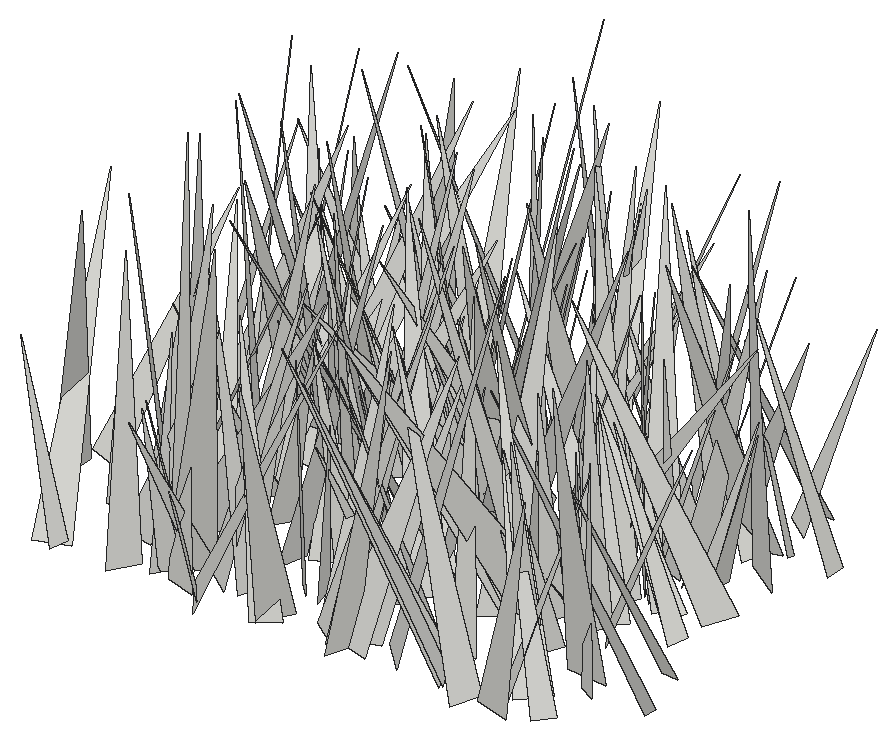
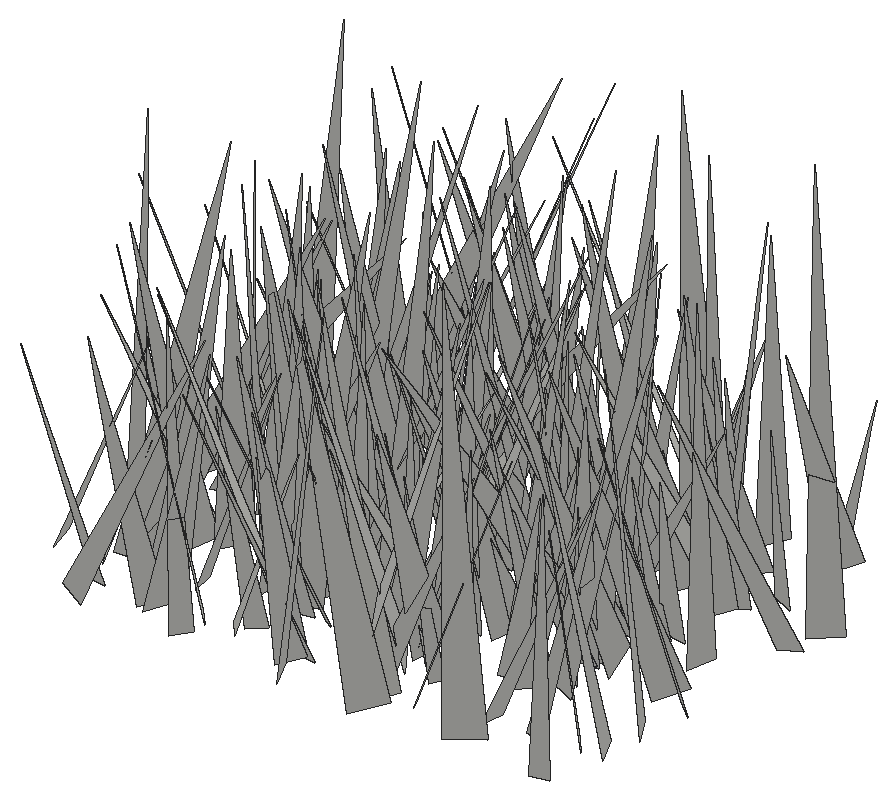
# SketchUp Ruby script. Lengths in inches.
U = 1.inch
M = Sketchup.active_model
def pt(a) = Geom::Point3d.new(a.map { |v| v * U })
def face(e, loops, mat)
  f = e.add_face(loops[0].map { |a| pt(a) })
  loops[1..].each { |l| e.add_face(l.map { |a| pt(a) }).erase! }
  f.material = f.back_material = mat if mat
  f
end
# faces: each face lists its corners as indices into pts; further lists are holes
def faces(e, pts, list, mat = nil) = list.each { |f| face(e, (f[0].is_a?(Array) ? f : [f]).map { |l| l.map { |i| pts[i] } }, mat) }
# xy, xz, yz: faces in a plane at the given z, y or x. An outline is a flat list of corners, or four numbers for a rectangle; further outlines are holes
def ring(l) = l.size == 4 ? [[l[0], l[1]], [l[2], l[1]], [l[2], l[3]], [l[0], l[3]]] : l.each_slice(2).to_a
def flat(e, list, mat, &to3) = list.each { |f| face(e, (f[0].is_a?(Array) ? f : [f]).map { |l| ring(l).map { |u, v| to3.(u, v) } }, mat) }
def xy(e, z, list, mat = nil) = flat(e, list, mat) { |x, y| [x, y, z] }
def xz(e, y, list, mat = nil) = flat(e, list, mat) { |x, z| [x, y, z] }
def yz(e, x, list, mat = nil) = flat(e, list, mat) { |y, z| [x, y, z] }
def lines(e, pts, list) = list.each { |a, b| e.add_line(pt(pts[a]), pt(pts[b])) }
# prism: a flat outline (further loops are holes) pulled along v
def prism(e, loops, v, mat = nil)
  f = face(e, loops, mat); d = Geom::Vector3d.new(v.map { |x| x * U })
  f.pushpull(f.normal.samedirection?(d) ? d.length : -d.length)
end
def box(e, o, s, mat = nil) = prism(e, [[o, [o[0] + s[0], o[1], o[2]], [o[0] + s[0], o[1] + s[1], o[2]], [o[0], o[1] + s[1], o[2]]]], [0, 0, s[2]], mat)
def at(x, y, z, deg = 0) = Geom::Transformation.translation(pt([x, y, z])) * Geom::Transformation.rotation(ORIGIN, Z_AXIS, deg.degrees)
def axes(o, x, y, z) = Geom::Transformation.new([*x, 0, *y, 0, *z, 0, *pt(o).to_a, 1])
def part(name) = M.definitions.add(name)
# library, detail: a bought-in or finely detailed component or shape, given as its bounding box
def library(name, o, s) = part(name).tap { |d| box(d.entities, o, s) }
def detail(e, o, s) = box(e.add_group.entities, o, s)
def put(e, d, t, mat = nil) = e.add_instance(d, t).tap { |i| i.material = mat if mat }
def group(e, t, mat = nil) = e.add_group.tap { |g| g.transformation = t; g.material = mat if mat }.entities
root = M.entities
c1 = part("fur_instance\#9")
p = [[0.8125,0,1.79],[0.67,-0.02,1.48],[0,-0.11,0],[0,0.11,0]]
faces(c1.entities,p,[[0,1,2,3]])
put(root,c1,axes([515.01,5.77,-21.86],[4.57924,-4.33247,0.58798],[-4.22206,-4.60304,-1.03525],[-1.13589,-0.35667,6.21836]))
put(root,c1,axes([521.93,6.4375,-21.86],[-6.83596,-2.73328,0.53057],[-2.58478,6.75268,1.48423],[1.035,-1.18879,7.21098]))
put(root,c1,axes([524.83,5.37,-21.86],[0.54307,-5.39112,1.14857],[-5.29865,-0.1925,1.60174],[1.51911,1.25582,5.17624]))
put(root,c1,axes([522.02,6.35,-21.86],[-5.72076,-3.26575,0.35826],[-3.1922,5.6955,0.94426],[0.77675,-0.64548,6.51924]))
put(root,c1,axes([510.13,6.12,-21.86],[2.18541,-3.04998,0.78828],[-3.02604,-2.29919,-0.50659],[-0.87571,0.3334,3.71777]))
put(root,c1,axes([511.02,6.96,-21.86],[1.51991,-3.61395,0.26794],[-3.4425,-1.53065,-1.11749],[-1.13207,-0.1975,3.75792]))
put(root,c1,axes([505.96,5.14,-21.86],[-3.79892,0.58903,0.61511],[0.5899,3.84804,-0.04166],[0.61427,-0.05255,3.84409]))
put(root,c1,axes([518.15,5.42,-21.86],[6.14943,-1.42717,1.61929],[-1.52874,-6.3314,0.22535],[-1.52376,0.59247,6.30885]))
put(root,c1,axes([510.14,7.22,-21.86],[6.18232,-5.30847,0.7026],[-5.32058,-6.21081,-0.10875],[-0.60412,0.37485,8.14795]))
put(root,c1,axes([511.93,5.12,-21.86],[5.9079,4.20697,0.32991],[4.15488,-5.69984,-1.72033],[0.73785,-1.5887,7.04573]))
put(root,c1,axes([512.08,5.14,-21.86],[-3.12705,-1.8127,0.50032],[-1.87769,2.95706,-1.02213],[-0.10232,1.13341,3.46693]))
put(root,c1,axes([508.7,5.31,-21.86],[-5.0872,2.66073,2.45988],[2.85923,5.55214,-0.09239],[2.22604,-1.05084,5.74025]))
put(root,c1,axes([514.94,5.33,-21.86],[-2.01026,5.06538,1.49078],[5.275,1.85579,0.80751],[-0.23431,-1.67916,5.38954]))
put(root,c1,axes([523.74,5.29,-21.86],[-6.69944,1.03913,0.45559],[1.00559,6.70154,-0.49804],[0.5255,0.42362,6.76123]))
put(root,c1,axes([517.66,5.93,-21.86],[5.24089,-0.83273,1.62957],[-1.05437,-5.41429,0.62423],[-1.49573,0.89885,5.2698]))
put(root,c1,axes([518.24,5.71,-21.86],[0.11042,6.13884,2.00494],[6.14565,0.51615,-1.91884],[1.98398,-1.94051,5.83229]))
put(root,c1,axes([503.14,9.33,-21.86],[8.00988,-2.00577,0.3429],[-1.833,-7.71682,-2.32157],[-0.88363,-2.17404,7.92412]))
put(root,c1,axes([511.07,5.46,-21.86],[2.99088,7.34321,2.70362],[7.47912,-3.53374,1.32409],[-2.30112,-1.94104,7.81761]))
put(root,c1,axes([526.625,5.99,-21.86],[-1.36293,4.52681,0.55653],[4.38086,1.13777,1.47406],[-1.26877,-0.93423,4.49185]))
put(root,c1,axes([509.84,5.78,-21.86],[-4.10668,0.43412,1.0008],[0.12519,4.05996,-1.24738],[1.0837,1.17608,3.93666]))
put(root,c1,axes([524.67,7.86,-21.86],[1.7038,-4.78318,1.39426],[-4.94528,-1.80274,-0.14134],[-0.60574,1.26373,5.0756]))
put(root,c1,axes([511.69,6.65,-21.86],[3.29943,5.39851,1.49465],[5.593,-3.07886,-1.22601],[0.31023,-1.9081,6.20701]))
put(root,c1,axes([525.93,9.21,-21.86],[0.64901,-7.30772,0.94418],[-7.33385,-0.54888,0.79295],[0.71332,1.00569,7.2935]))
put(root,c1,axes([524.82,5.97,-21.86],[3.07177,3.42083,0.35758],[3.42072,-3.08846,0.16062],[-0.35863,-0.15826,4.59478]))
put(root,c1,axes([519.84,6.17,-21.86],[5.42391,5.6075,1.42758],[5.74422,-5.4537,-0.40246],[-0.69711,-1.3092,7.79108]))
put(root,c1,axes([507.74,7.23,-21.86],[1.80806,-4.3936,1.6396],[-4.55829,-1.23367,1.72079],[1.10181,2.10605,4.4285]))
put(root,c1,axes([515.34,8,-21.86],[3.69206,0.52175,1.19179],[0.74035,-3.79133,-0.63373],[-1.0698,-0.8231,3.6745]))
put(root,c1,axes([520.88,7.52,-21.86],[-4.50374,-2.5863,0.2222],[-2.55985,4.35118,-1.23954],[-0.43072,1.18335,5.04343]))
put(root,c1,axes([522.21,11.63,-21.86],[4.91107,-6.51993,1.1851],[-5.42781,-4.80392,-3.93621],[-3.80168,-1.5638,7.15082]))
put(root,c1,axes([513.12,6.66,-21.86],[-5.72971,0.10944,0.75393],[-0.02545,5.68949,-1.01935],[0.7614,1.01378,5.63937]))
put(root,c1,axes([517.03,5.94,-21.86],[4.48947,6.23838,0.89691],[6.27438,-4.52789,0.08708],[-0.59503,-0.67674,7.68539]))
put(root,c1,axes([507.99,8.89,-21.86],[-4.21383,-5.23135,2.06774],[-5.35043,4.52497,0.54449],[1.7365,1.24763,6.69529]))
put(root,c1,axes([525.42,6.91,-21.86],[-3.60307,5.2202,0.86904],[5.28801,3.51043,0.83765],[-0.20649,-1.18922,6.28736]))
put(root,c1,axes([517.56,9.05,-21.86],[0.6602,-3.48398,0.63366],[-3.31771,-0.83389,-1.12823],[-1.23791,0.37685,3.36171]))
put(root,c1,axes([505.6875,5.11,-21.86],[-5.02723,4.35262,0.08247],[4.19421,4.87628,-1.68986],[1.1665,1.22544,6.43138]))
put(root,c1,axes([514.53,7.9375,-21.86],[2.78644,2.89477,1.9564],[3.12581,-3.18339,0.25829],[-1.56092,-1.20736,4.00964]))
put(root,c1,axes([516.08,8.74,-21.86],[2.18387,-4.44969,1.85832],[-4.59717,-2.53702,-0.67228],[-1.45572,1.33648,4.91091]))
put(root,c1,axes([518.57,6.35,-21.86],[-3.94538,2.89092,1.6801],[2.22143,4.20848,-2.02488],[2.49909,0.82308,4.45234]))
put(root,c1,axes([516.7,6.97,-21.86],[0.1573,5.82785,1.1486],[5.93788,-0.12389,-0.18455],[0.15705,-1.15268,5.82705]))
put(root,c1,axes([516.33,7.68,-21.86],[6.01682,-1.89651,1.60783],[-2.22,-5.99358,1.23799],[-1.11958,1.69241,6.18597]))
put(root,c1,axes([526.65,8.32,-21.86],[2.05844,3.54151,1.67651],[3.74882,-2.33096,0.32115],[-1.13989,-1.27062,4.08367]))
put(root,c1,axes([523.8,9.9,-21.86],[3.25434,-3.10316,1.28908],[-2.93626,-3.49873,-1.00964],[-1.63392,0.10675,4.38189]))
put(root,c1,axes([508.94,9.32,-21.86],[3.69144,-5.31541,0.62902],[-5.0613,-3.21782,2.51095],[1.74141,1.9152,5.96452]))
put(root,c1,axes([521.02,11.38,-21.86],[-6.06549,-1.51995,0.44377],[-1.27134,5.72216,2.22212],[0.94386,-2.06007,5.84487]))
put(root,c1,axes([529.18,8.63,-21.86],[-3.79929,-4.93063,0.76728],[-4.2284,2.66909,-3.78564],[-2.64961,2.81057,4.94112]))
put(root,c1,axes([505.8,8.41,-21.86],[0.89714,3.83975,1.01573],[3.88067,-1.06922,0.61438],[-0.84607,-0.83267,3.89501]))
put(root,c1,axes([506.81,9.65,-21.86],[1.60896,-4.17155,1.4473],[-4.41412,-1.4813,0.63763],[0.1098,1.57772,4.42538]))
put(root,c1,axes([521.68,7.73,-21.86],[1.15539,6.15443,1.22459],[6.01284,-1.44203,1.57415],[-1.79512,-0.86897,6.06086]))
put(root,c1,axes([515.49,9.5,-21.86],[2.89079,5.81329,3.19782],[6.3896,-3.37876,0.3661],[-1.787,-2.67707,6.48205]))
put(root,c1,axes([528.125,11.05,-21.86],[-1.33885,-4.31341,0.19295],[-4.24788,1.27969,-0.86785],[-0.77346,0.43835,4.43226]))
put(root,c1,axes([522.77,10.72,-21.86],[-7.92829,-1.68885,1.19775],[-1.65667,8.01779,0.33921],[1.24187,-0.08605,8.09907]))
put(root,c1,axes([519.47,10.6,-21.86],[-4.42248,-6.55022,0.11235],[-5.68971,3.77318,-3.9833],[-3.24733,2.30957,6.8262]))
put(root,c1,axes([512.99,9.21,-21.86],[6.83211,0.09479,1.62922],[-0.11306,-6.96812,0.87954],[-1.62805,0.88169,6.77592]))
put(root,c1,axes([510.66,9.52,-21.86],[6.64236,-2.17739,2.19825],[-2.53423,-6.81539,0.90685],[-1.77512,1.5823,6.93106]))
put(root,c1,axes([515.02,12.3,-21.86],[-2.64137,-6.46023,1.04071],[-6.35863,2.79897,1.23619],[1.54452,0.47506,6.86901]))
put(root,c1,axes([516.75,10.65,-21.86],[-2.99975,-3.60869,1.08185],[-3.74003,3.01886,-0.30041],[0.45307,1.02732,4.68304]))
put(root,c1,axes([517.97,11.37,-21.86],[-2.72161,-4.19987,1.18368],[-4.18397,2.90781,0.69726],[1.23872,0.59401,4.95579]))
put(root,c1,axes([517.01,11.89,-21.86],[-3.4454,-3.89131,0.03074],[-3.88746,3.44363,0.20759],[0.17579,-0.11462,5.19326]))
put(root,c1,axes([507.0625,10.29,-21.86],[5.24676,-2.59436,1.90695],[-2.83441,-5.4512,0.38233],[-1.5275,1.20389,5.84064]))
put(root,c1,axes([511.02,11.1,-21.86],[3.98619,-2.41358,0.43201],[-2.42835,-4.00018,0.05811],[-0.33929,0.27366,4.65958]))
put(root,c1,axes([525.1,9.96,-21.86],[-3.3024,-1.44134,1.34219],[-1.74105,3.36144,-0.674],[0.92071,1.18661,3.53964]))
put(root,c1,axes([513.57,11.0625,-21.86],[-4.43723,-6.45792,2.6794],[-6.95056,4.4181,-0.86196],[0.75734,2.71083,7.78786]))
put(root,c1,axes([518.09,10.12,-21.86],[-4.29093,5.93832,1.73067],[6.14946,4.32229,0.41585],[0.66564,-1.65078,7.31456]))
put(root,c1,axes([522.53,11.625,-21.86],[3.95695,-1.9726,1.7752],[-1.97238,-4.31833,-0.40205],[-1.77544,0.40099,4.40306]))
put(root,c1,axes([518.07,10.95,-21.86],[3.90442,0.1948,1.09665],[0.0575,-4.02752,0.51071],[-1.11233,0.47558,3.87577]))
put(root,c1,axes([507.72,9.43,-21.86],[5.65943,2.62486,0.30549],[2.50558,-5.55953,1.3513],[-0.8398,1.10185,6.0904]))
put(root,c1,axes([509.74,12.45,-21.86],[-0.92246,-4.02488,0.49642],[-3.83236,0.69867,-1.45667],[-1.32631,0.78053,3.86377]))
put(root,c1,axes([524.09,11.98,-21.86],[4.08918,-3.36848,1.98263],[-3.52303,-4.41912,-0.24183],[-1.69286,1.05996,5.29241]))
put(root,c1,axes([512.59,13.29,-21.86],[2.722,-4.21365,0.18087],[-4.20663,-2.72794,-0.24377],[-0.30292,0.01939,5.01046]))
put(root,c1,axes([524.68,11.875,-21.86],[4.18709,2.7222,0.51054],[2.74144,-3.94162,-1.4666],[0.39441,-1.502,4.77401]))
put(root,c1,axes([518.31,10.74,-21.86],[-4.785,3.6619,0.62252],[3.69492,4.79647,0.18627],[0.38032,-0.52686,6.02254]))
put(root,c1,axes([520.21,14.44,-21.86],[-1.4202,-8.16889,0.91065],[-8.13373,1.52988,1.03868],[1.18423,0.71114,8.22611]))
put(root,c1,axes([510.73,10.49,-21.86],[-6.74078,-2.87477,2.26806],[-3.46071,6.55422,-1.97791],[1.19661,2.76122,7.05622]))
put(root,c1,axes([517.1,12.01,-21.86],[-5.1041,-1.8904,0.52095],[-1.9461,5.06157,-0.70004],[0.24022,0.83889,5.39772]))
put(root,c1,axes([523.39,13,-21.86],[3.43553,-2.13589,0.95207],[-2.02418,-3.56342,-0.68999],[-1.17096,-0.10667,3.98608]))
put(root,c1,axes([513.78,9.9,-21.86],[-4.67511,2.29396,0.21165],[2.12082,4.47274,-1.63107],[0.89953,1.37696,4.94555]))
put(root,c1,axes([520.89,10.65,-21.86],[5.55139,-3.03279,3.66915],[-4.09539,-5.91606,1.30628],[-2.42657,3.04644,6.18946]))
put(root,c1,axes([519.7,13.21,-21.86],[-3.40896,-3.60182,1.17644],[-3.63778,3.55381,0.3393],[1.06005,0.61272,4.94762]))
put(root,c1,axes([503.53,10.8,-21.86],[0.65579,5.75921,0.77226],[5.58682,-0.41126,-1.67728],[1.5976,-0.92592,5.54845]))
put(root,c1,axes([514.83,10.61,-21.86],[3.66563,6.83822,1.35122],[6.90712,-3.76874,0.33492],[-0.93742,-1.02919,7.75151]))
put(root,c1,axes([515.43,17.06,-21.86],[-6.54697,-3.05595,0.68846],[-2.14459,5.53525,4.1758],[2.28332,-3.56338,5.89613]))
put(root,c1,axes([508.72,12.56,-21.86],[2.49544,-4.2024,1.5625],[-4.46283,-2.15679,1.32672],[0.42981,2.0042,4.70396]))
put(root,c1,axes([511.19,13.94,-21.86],[4.7247,0.27251,1.48983],[0.66278,-4.76043,-1.23114],[-1.36183,-1.37139,4.56961]))
put(root,c1,axes([505.3,13.47,-21.86],[6.40054,-0.55178,2.21578],[-0.37829,-6.75939,-0.5905],[-2.25189,-0.43282,6.39709]))
put(root,c1,axes([508.59,15.75,-21.86],[2.6634,-7.09113,0.13913],[-7.08626,-2.66678,-0.26525],[-0.29724,0.03689,7.57017]))
put(root,c1,axes([524.43,12.79,-21.86],[-1.64307,3.38565,0.94063],[3.51296,1.55882,0.52563],[-0.08077,-1.0745,3.72639]))
put(root,c1,axes([526.84,13.06,-21.86],[-3.98782,0.86871,0.11292],[0.87287,3.98492,0.16912],[0.07423,-0.18933,4.07783]))
put(root,c1,axes([517.34,15.29,-21.86],[4.0127,-3.86264,0.72099],[-3.71726,-4.06564,-1.09277],[-1.27351,-0.30356,5.46147]))
put(root,c1,axes([511.84,14.54,-21.86],[-1.12963,-3.6746,0.26296],[-3.62855,1.06225,-0.74377],[-0.63679,0.46567,3.77168]))
put(root,c1,axes([517.87,17.13,-21.86],[-6.83742,-2.67371,1.15288],[-1.91772,6.34944,3.35188],[2.19094,-2.7864,6.53176]))
put(root,c1,axes([516.02,17.06,-21.86],[7.80685,-2.34529,0.78759],[-1.91376,-7.37702,-2.99744],[-1.56786,-2.67335,7.58041]))
put(root,c1,axes([507.5625,12.85,-21.86],[0.0321,3.78164,0.61426],[3.82721,-0.05969,0.16749],[-0.17489,-0.6122,3.77806]))
put(root,c1,axes([521.64,11.81,-21.86],[5.08694,2.79276,1.06084],[2.31416,-5.00849,2.08845],[-1.88933,1.38471,5.41433]))
put(root,c1,axes([514.43,15.92,-21.86],[-4.64993,-4.92524,0.42817],[-4.93518,4.6591,-0.00251],[0.29211,0.31306,6.77347]))
put(root,c1,axes([527.07,15.12,-21.86],[-3.6368,4.97548,2.15784],[5.29036,2.68314,2.72961],[-1.1932,-3.26854,5.52548]))
put(root,c1,axes([525.71,14.29,-21.86],[-3.19624,2.75407,0.40141],[2.73336,2.9911,1.24258],[-0.52417,-1.19599,4.03198]))
put(root,c1,axes([507.27,12.6,-21.86],[-0.56854,4.75375,0.07359],[4.64609,0.5398,1.02436],[-1.0087,-0.19303,4.67676]))
put(root,c1,axes([523.3,15.65,-21.86],[-4.22534,-4.50008,2.6097],[-4.33201,4.90527,1.44456],[2.88009,0.77613,6.00146]))
put(root,c1,axes([518.49,14.35,-21.86],[6.91635,-1.96319,0.7746],[-2.05636,-6.86586,0.95992],[-0.47486,1.1384,7.12521]))
put(root,c1,axes([517.42,13.93,-21.86],[7.84011,2.17766,1.89393],[2.14429,-8.06482,0.39652],[-1.93163,-0.114,8.12726]))
put(root,c1,axes([518.125,14.63,-21.86],[-4.47703,-2.46915,0.00102],[-2.34184,4.24552,-1.62229],[-0.78262,1.42103,4.84857]))
put(root,c1,axes([509.39,14.85,-21.86],[5.44742,2.57642,1.57153],[2.74581,-5.57692,-0.37485],[-1.25227,-1.0208,6.0143]))
put(root,c1,axes([523.59,13.92,-21.86],[-7.28379,2.71503,1.56111],[2.64145,7.44897,-0.63058],[1.68261,0.05921,7.74773]))
put(root,c1,axes([522.57,15.79,-21.86],[5.81902,2.09502,1.94943],[2.48849,-5.88572,-1.1028],[-1.4131,-1.7377,6.08555]))
put(root,c1,axes([513.9,14.45,-21.86],[0.71871,3.7725,0.80138],[3.83913,-0.62217,-0.51422],[0.36739,-0.87844,3.80576]))
put(root,c1,axes([508.6875,13.49,-21.86],[1.55452,5.85258,0.28483],[5.77094,-1.47817,-1.12324],[1.01494,-0.55917,5.95042]))
put(root,c1,axes([516.14,15.97,-21.86],[0.22689,-3.51122,0.97081],[-3.62685,-0.12635,0.39066],[0.3422,0.98893,3.49679]))
put(root,c1,axes([522.58,14.67,-21.86],[-2.56552,5.11443,0.44811],[4.78646,2.20153,2.27666],[-1.85689,-1.39139,5.24939]))
put(root,c1,axes([514.09,15.05,-21.86],[2.7927,4.03544,0.85961],[4.11922,-2.66751,-0.85986],[0.23622,-1.19268,4.83163]))
put(root,c1,axes([510.59,17.125,-21.86],[-2.6676,-6.3456,1.58153],[-6.4273,2.85927,0.63121],[1.20736,1.20081,6.85451]))
put(root,c1,axes([525.12,14.48,-21.86],[-0.96186,4.58475,0.31518],[4.19254,0.74357,1.97843],[-1.88199,-0.68675,4.24628]))
put(root,c1,axes([523.36,12.9,-21.86],[-7.41355,2.38035,1.13819],[1.92535,7.2016,-2.52036],[1.80404,2.09598,7.36713]))
put(root,c1,axes([525.7,15.55,-21.86],[1.6531,3.56586,0.9383],[3.65871,-1.45863,-0.90264],[0.45784,-1.21883,3.82535]))
put(root,c1,axes([511.46,15.26,-21.86],[-0.23432,4.6061,1.3303],[4.44797,-0.2882,1.78136],[-1.78924,-1.31967,4.25416]))
put(root,c1,axes([520.12,17.26,-21.86],[5.88193,4.68919,0.48239],[4.10623,-4.71789,-4.20698],[2.31519,-3.54559,6.23594]))
put(root,c1,axes([514.85,16.18,-21.86],[-3.89073,-0.42692,0.42553],[-0.44504,3.90915,-0.14719],[0.40654,0.19356,3.91132]))
put(root,c1,axes([523.68,16.66,-21.86],[-0.96334,-4.21277,1.52504],[-4.43315,1.12201,0.29911],[0.64835,1.41239,4.31115]))
put(root,c1,axes([521.76,15.3,-21.86],[-5.3119,3.70536,1.5571],[3.75007,5.49761,-0.28937],[1.44609,-0.64586,6.4701]))
put(root,c1,axes([519.51,15.74,-21.86],[-4.33935,-4.28478,3.74469],[-5.00881,5.11096,0.04388],[2.70071,2.59437,6.09815]))
put(root,c1,axes([524.06,14.89,-21.86],[3.70568,3.40586,0.49894],[3.35111,-3.73706,0.62078],[-0.78668,0.12425,4.99466]))
put(root,c1,axes([508.03,17.85,-21.86],[-2.53564,-6.45433,1.27855],[-6.57975,2.48748,-0.49186],[0.00081,1.3699,6.91708]))
put(root,c1,axes([525.52,16.99,-21.86],[3.83276,-0.80553,0.30542],[-0.78769,-3.84079,-0.24507],[-0.34886,-0.17786,3.90882]))
put(root,c1,axes([510.99,15.71,-21.86],[0.50211,5.33526,1.29674],[5.04367,0.06639,-2.22613],[2.16978,-1.38897,4.87457]))
put(root,c1,axes([504.77,15.8,-21.86],[4.48664,-4.30175,1.96808],[-4.72578,-3.95369,2.13158],[0.21294,2.89338,5.83878]))
put(root,c1,axes([518.26,15.17,-21.86],[-6.64988,-1.58039,2.79885],[-2.32051,6.81074,-1.66765],[2.22405,2.38079,6.62853]))
put(root,c1,axes([518.65,18.79,-21.86],[2.5513,-6.67742,1.15565],[-6.68995,-2.67869,-0.70836],[-1.08074,0.81812,7.11304]))
put(root,c1,axes([525.11,19.83,-21.86],[1.39715,-7.46285,0.32526],[-7.45597,-1.41344,-0.40331],[-0.45656,0.24497,7.58179]))
put(root,c1,axes([511.85,15.86,-21.86],[-4.5359,3.17744,2.60533],[2.766,5.23085,-1.56386],[3.0386,-0.01843,5.3127]))
put(root,c1,axes([513.91,18.01,-21.86],[-4.72321,-4.87597,2.05821],[-5.0831,4.94763,0.05633],[1.47426,1.43735,6.78828]))
put(root,c1,axes([503.8,16.29,-21.86],[3.62165,4.35293,0.90177],[4.41878,-3.65214,-0.11732],[-0.48531,-0.76904,5.66132]))
put(root,c1,axes([513.16,16.89,-21.86],[-2.98056,5.41129,1.99239],[5.72855,3.03527,0.32601],[0.65987,-1.90801,6.16924]))
put(root,c1,axes([526.35,18.35,-21.86],[3.79237,5.90894,3.79832],[6.9076,-3.92109,-0.79686],[-1.27587,-3.6653,6.97586]))
put(root,c1,axes([514.63,16.97,-21.86],[-0.71726,5.0627,1.58469],[5.02661,0.13746,1.836],[-1.69568,-1.73401,4.77227]))
put(root,c1,axes([508.56,15.91,-21.86],[2.2285,7.10603,0.93052],[7.02267,-1.97084,-1.76797],[1.42959,-1.39565,7.23438]))
put(root,c1,axes([508.22,16.84,-21.86],[2.91004,3.86675,2.0314],[3.84438,-3.42612,1.0144],[-2.0734,-0.92551,4.73192]))
put(root,c1,axes([518.43,18.21,-21.86],[6.40795,-1.734,1.03011],[-1.73088,-6.48917,-0.15614],[-1.03535,0.11648,6.63658]))
put(root,c1,axes([507.59,15.13,-21.86],[-6.44163,0.17845,3.84936],[-1.24896,6.99677,-2.4144],[3.64548,2.71245,5.9747]))
put(root,c1,axes([508.71,15.97,-21.86],[-2.09458,6.39775,0.76013],[6.40195,1.97698,1.00139],[-0.72385,-1.02792,6.657]))
put(root,c1,axes([514.06,17.68,-21.86],[-7.0839,-2.86843,1.00142],[-2.98784,7.03787,-0.97651],[0.55097,1.28563,7.57997]))
put(root,c1,axes([508.73,14.87,-21.86],[-2.61013,7.00123,1.33294],[6.01827,2.92557,-3.58165],[3.81765,0.17478,6.55758]))
put(root,c1,axes([523.98,17.6,-21.86],[5.79665,-1.91222,1.6292],[-2.17494,-5.87047,0.84811],[-1.25719,1.33905,6.04471]))
put(root,c1,axes([508.91,17.63,-21.86],[0.82444,4.69785,1.50621],[4.90559,-0.61872,-0.75536],[0.52313,-1.60174,4.70945]))
put(root,c1,axes([523,16.99,-21.86],[-5.28353,4.19242,1.51467],[4.2139,5.46353,-0.42331],[1.45386,-0.59977,6.73148]))
put(root,c1,axes([514.93,18.12,-21.86],[-6.49588,1.72746,1.45223],[1.82521,6.62397,0.28488],[1.32729,-0.65455,6.71561]))
put(root,c1,axes([516.6875,16.62,-21.86],[3.32895,2.2471,0.95718],[1.81279,-3.35751,1.57751],[-1.63691,0.85163,3.69362]))
put(root,c1,axes([517.75,16.76,-21.86],[1.80048,6.74236,1.9451],[6.61582,-2.30046,1.85022],[-2.33959,-1.31645,6.72888]))
put(root,c1,axes([514.66,16.41,-21.86],[4.4552,2.25801,0.37031],[2.04407,-4.29173,1.57715],[-1.02836,1.2518,4.7392]))
put(root,c1,axes([503.99,18.37,-21.86],[5.69134,3.55142,2.30083],[3.82093,-5.97012,-0.23634],[-1.81848,-1.42926,6.70433]))
put(root,c1,axes([524.43,16.41,-21.86],[4.78963,3.34115,0.62659],[3.09789,-4.73577,1.57225],[-1.39963,0.95165,5.62422]))
put(root,c1,axes([515.68,19.375,-21.86],[4.61843,1.91697,0.98697],[2.11588,-4.47821,-1.2031],[-0.41467,-1.49987,4.85358]))
put(root,c1,axes([509.05,18.64,-21.86],[-3.73085,2.02538,0.45172],[2.07172,3.68874,0.57157],[0.11914,-0.71871,4.20651]))
put(root,c1,axes([509.77,18.34,-21.86],[-1.66438,3.94539,0.96796],[4.04045,1.49913,0.83702],[-0.42169,-1.20819,4.19948]))
put(root,c1,axes([512.83,19.11,-21.86],[3.65523,2.01923,0.98653],[2.16689,-3.66612,-0.52479],[-0.59594,-0.94526,4.14277]))
put(root,c1,axes([513.86,17.66,-21.86],[6.24718,3.3719,1.68528],[3.2403,-6.4703,0.93425],[-1.92623,0.05148,7.03734]))
put(root,c1,axes([506.56,21.04,-21.86],[-1.82022,-4.66244,0.24993],[-4.60062,1.83672,0.75812],[0.79693,-0.04591,4.9474]))
put(root,c1,axes([522.23,19.73,-21.86],[-4.58656,-0.99691,0.53395],[-0.9871,4.61746,0.14195],[0.55187,-0.02624,4.69151]))
put(root,c1,axes([511.65,20.08,-21.86],[3.62629,-0.3933,0.08931],[-0.3696,-3.56406,-0.68808],[-0.16141,-0.67481,3.58206]))
put(root,c1,axes([525.17,19.29,-21.86],[-3.66432,1.46778,0.50332],[1.5223,3.65057,0.437],[0.30055,-0.59495,3.9231]))
put(root,c1,axes([523.2,20.5,-21.86],[1.6386,-6.2759,2.07036],[-6.47654,-1.94928,-0.78297],[-1.31443,1.78093,6.43885]))
put(root,c1,axes([517.08,19.24,-21.86],[3.37481,3.69249,0.11879],[3.55193,-3.19874,-1.47981],[1.01606,-1.08238,4.77849]))
put(root,c1,axes([513.52,20.66,-21.86],[-0.67131,-4.1889,0.93111],[-4.10147,0.34927,-1.38579],[-1.26165,1.09345,4.00962]))
put(root,c1,axes([511.26,21.74,-21.86],[-4.05728,-2.523,0.42943],[-2.40041,4.03064,1.00168],[0.88766,-0.63233,4.67158]))
put(root,c1,axes([520.24,18.27,-21.86],[-7.28792,0.99409,0.70676],[0.80322,7.1337,-1.75122],[0.9179,1.65037,7.1439]))
put(root,c1,axes([513.68,22.34,-21.86],[-5.81753,-5.50464,0.89808],[-5.45533,5.88597,0.73893],[1.16061,0.07452,7.97488]))
put(root,c1,axes([516.14,17.79,-21.86],[3.59429,3.23742,0.8797],[2.57384,-3.488,2.32011],[-2.15177,1.23558,4.24464]))
put(root,c1,axes([509.66,21.15,-21.86],[4.3427,-1.50818,1.19732],[-1.3579,-4.49272,-0.73402],[-1.36538,-0.32877,4.53816]))
put(root,c1,axes([508.51,20.98,-21.86],[-5.398,0.07669,0.31538],[0.11355,5.36878,0.63804],[0.30406,-0.64352,5.36071]))
put(root,c1,axes([512.35,21.98,-21.86],[7.393,0.04175,0.28729],[0.1077,-7.1937,-1.72622],[-0.26959,-1.72907,7.18877]))
put(root,c1,axes([528.02,20.25,-21.86],[-5.12979,-1.0122,0.11272],[-1.018,5.07872,-0.72273],[-0.03042,0.73083,5.17851]))
put(root,c1,axes([508.37,22.64,-21.86],[2.3597,-7.64104,0.82634],[-7.58316,-2.17409,1.55097],[1.25061,1.23463,7.84527]))
put(root,c1,axes([505,20.5,-21.86],[3.09566,2.75124,1.27433],[2.88928,-3.22895,-0.04754],[-0.91941,-0.88367,4.14127]))
put(root,c1,axes([504.07,20.22,-21.86],[5.547,2.87669,1.51326],[2.93945,-5.71712,0.09337],[-1.38744,-0.61131,6.24786]))
put(root,c1,axes([518.81,21.02,-21.86],[-0.37702,3.57753,2.02822],[3.88687,0.97529,-0.99777],[1.34335,-1.81786,3.4562]))
put(root,c1,axes([526.13,20.19,-21.86],[-3.59352,-1.36236,0.30323],[-1.35819,3.22059,-1.62619],[-0.32136,1.6227,3.48208]))
put(root,c1,axes([519.4,21.52,-21.86],[-2.83398,-2.56318,0.53676],[-2.6174,2.79801,-0.45803],[0.08496,0.70049,3.79362]))
put(root,c1,axes([522.71,21.91,-21.86],[3.4493,-3.36014,0.02886],[-3.29462,-3.37365,0.97621],[0.66096,0.719,4.71542]))
put(root,c1,axes([520.61,22.92,-21.86],[5.40312,-1.02873,0.51523],[-0.87968,-5.28821,-1.33359],[-0.74156,-1.2223,5.33606]))
put(root,c1,axes([518.37,19.51,-21.86],[-5.21181,1.32812,1.31914],[0.83689,5.14396,-1.87252],[1.67442,1.56295,5.04188]))
put(root,c1,axes([513.14,18.49,-21.86],[-5.92228,3.52878,0.304],[3.26745,5.67188,-2.1844],[1.36692,1.73077,6.53866]))
put(root,c1,axes([517.12,20.97,-21.86],[6.15209,3.35933,0.33959],[3.37614,-6.1107,-0.71393],[0.04606,-0.78923,6.97306]))
put(root,c1,axes([525.28,23.1,-21.86],[-1.88046,-5.21634,0.33238],[-5.10911,1.75978,-1.28722],[-1.10347,0.74146,5.39346]))
put(root,c1,axes([520.7,21.57,-21.86],[5.36031,4.39922,1.5205],[4.6383,-5.24227,-1.18439],[-0.38885,-1.88772,6.83252]))
put(root,c1,axes([522.39,22.07,-21.86],[-5.09295,0.86723,1.4086],[1.03106,5.23004,0.50795],[1.29351,-0.75432,5.14123]))
put(root,c1,axes([513.56,19.35,-21.86],[6.37842,4.90538,1.53696],[4.59516,-6.53882,1.79932],[-2.30422,0.53885,7.84279]))
put(root,c1,axes([518.48,19.37,-21.86],[-1.83957,6.80237,0.25254],[6.80704,1.83779,0.08208],[-0.01336,-0.2652,7.04624]))
put(root,c1,axes([504.6875,23.16,-21.86],[-0.50328,-4.91347,1.0032],[-4.85841,0.72759,1.12622],[1.24277,0.85458,4.80907]))
put(root,c1,axes([512.3,23.01,-21.86],[6.42408,-3.63909,0.41323],[-3.66082,-6.40525,0.50369],[-0.11006,0.64215,7.36601]))
put(root,c1,axes([516.01,21.62,-21.86],[2.98745,4.37857,0.43851],[4.21633,-2.69647,-1.80015],[1.25963,-1.35874,4.98559]))
put(root,c1,axes([525.04,21.91,-21.86],[2.35379,3.88662,0.95748],[3.9563,-2.09005,-1.24191],[0.60851,-1.44527,4.3708]))
put(root,c1,axes([516.45,22.06,-21.86],[4.29417,-2.87763,1.75823],[-3.19183,-4.38696,0.6155],[-1.08829,1.5119,5.13243]))
put(root,c1,axes([516.1875,22.95,-21.86],[-6.04607,-3.24149,2.31572],[-3.3744,6.40425,0.15438],[2.11738,0.95032,6.85845]))
